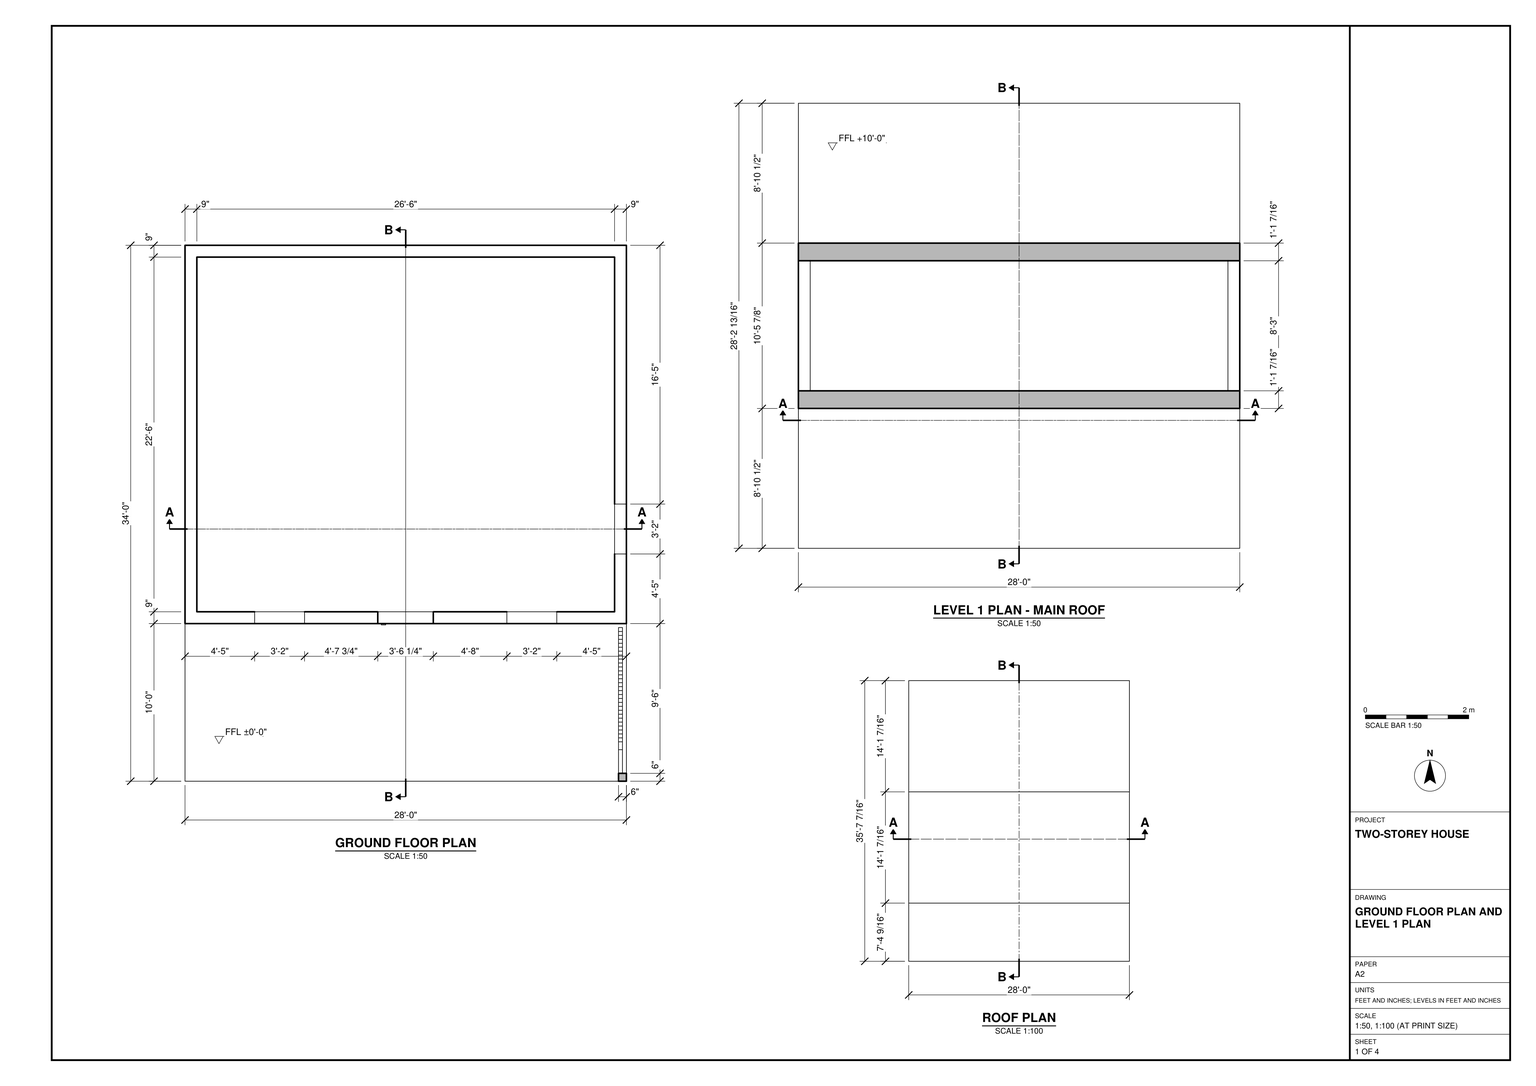
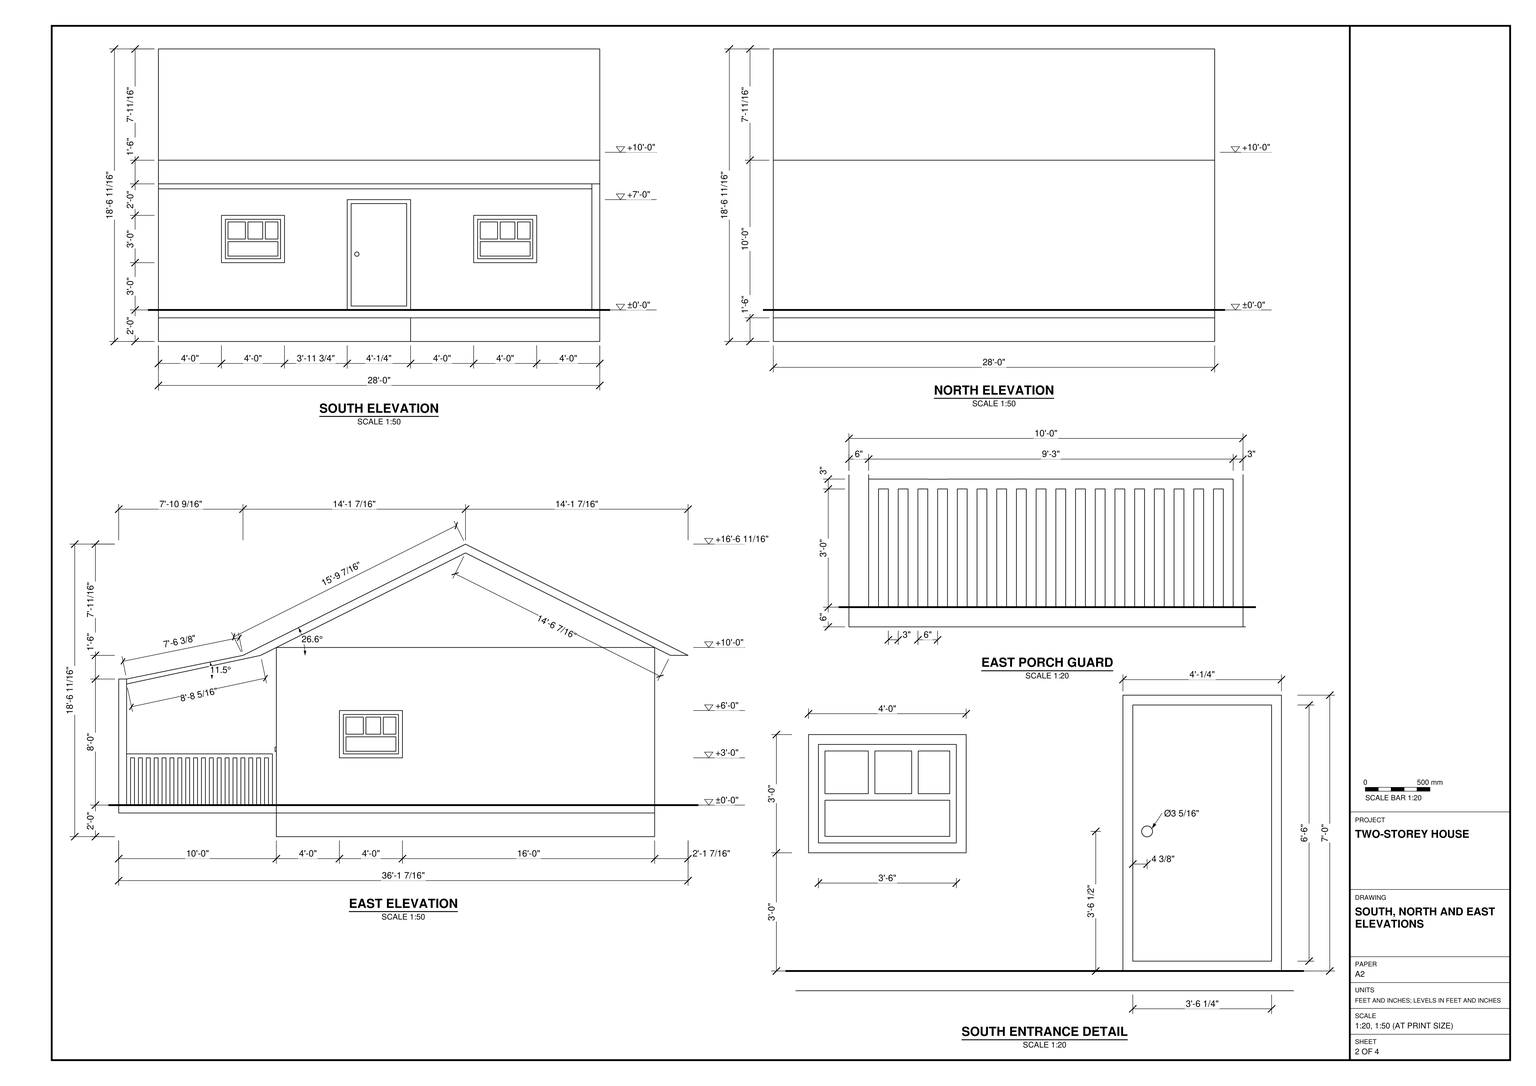
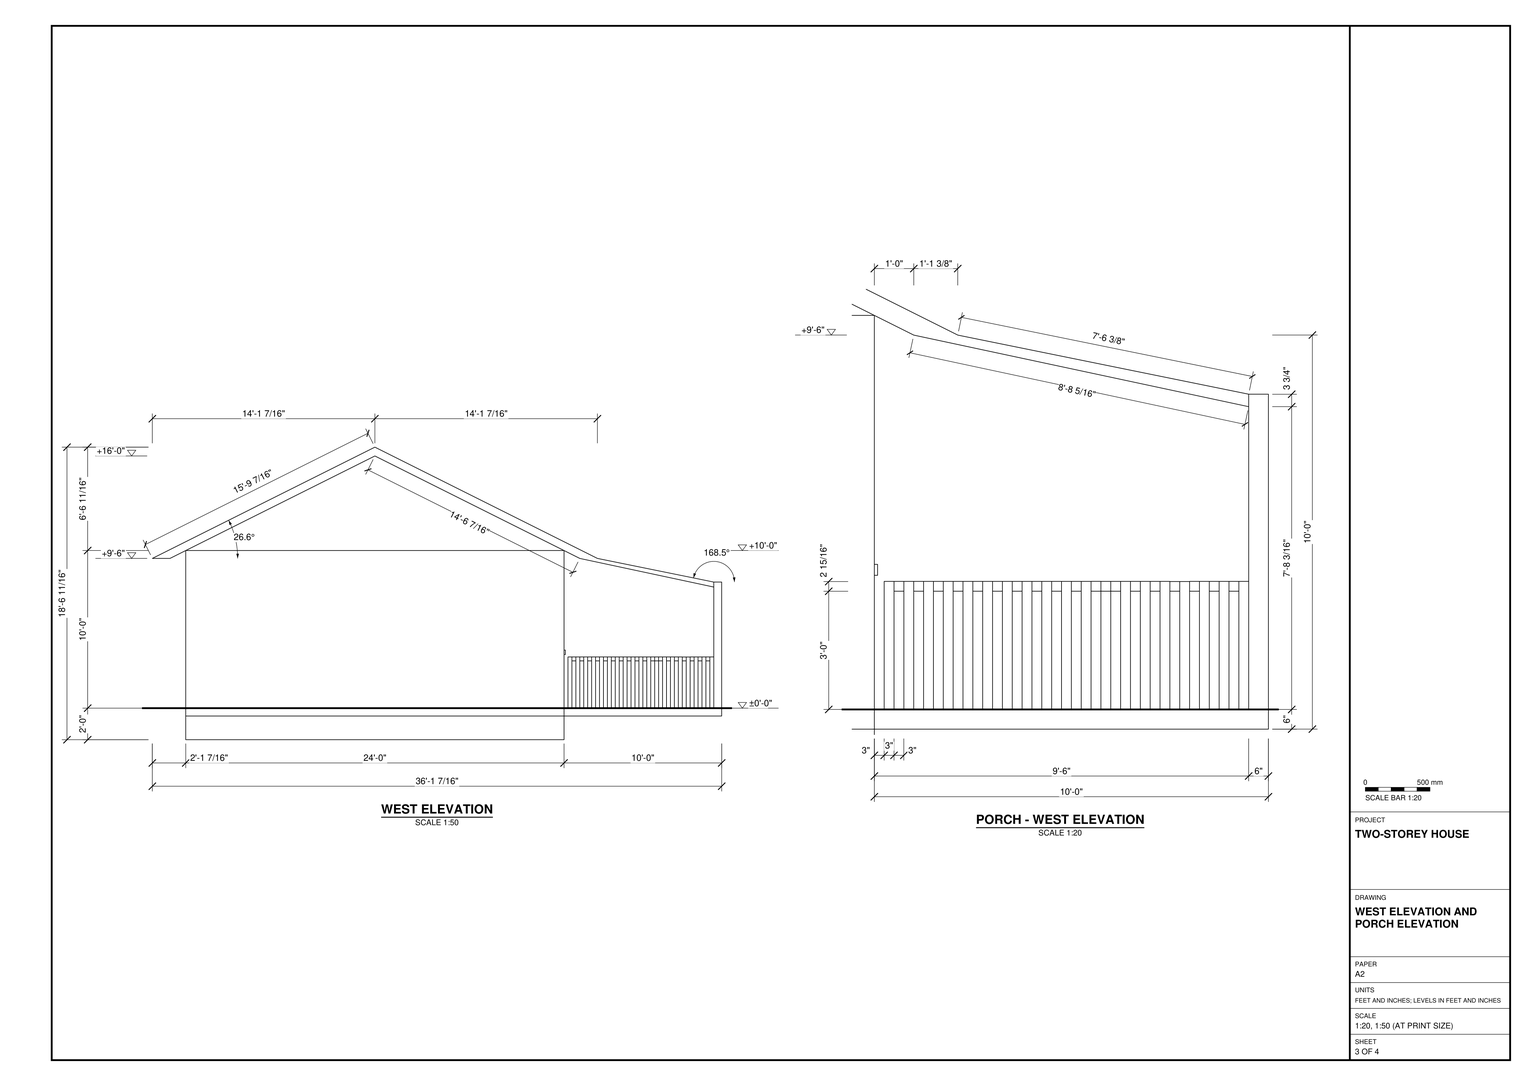
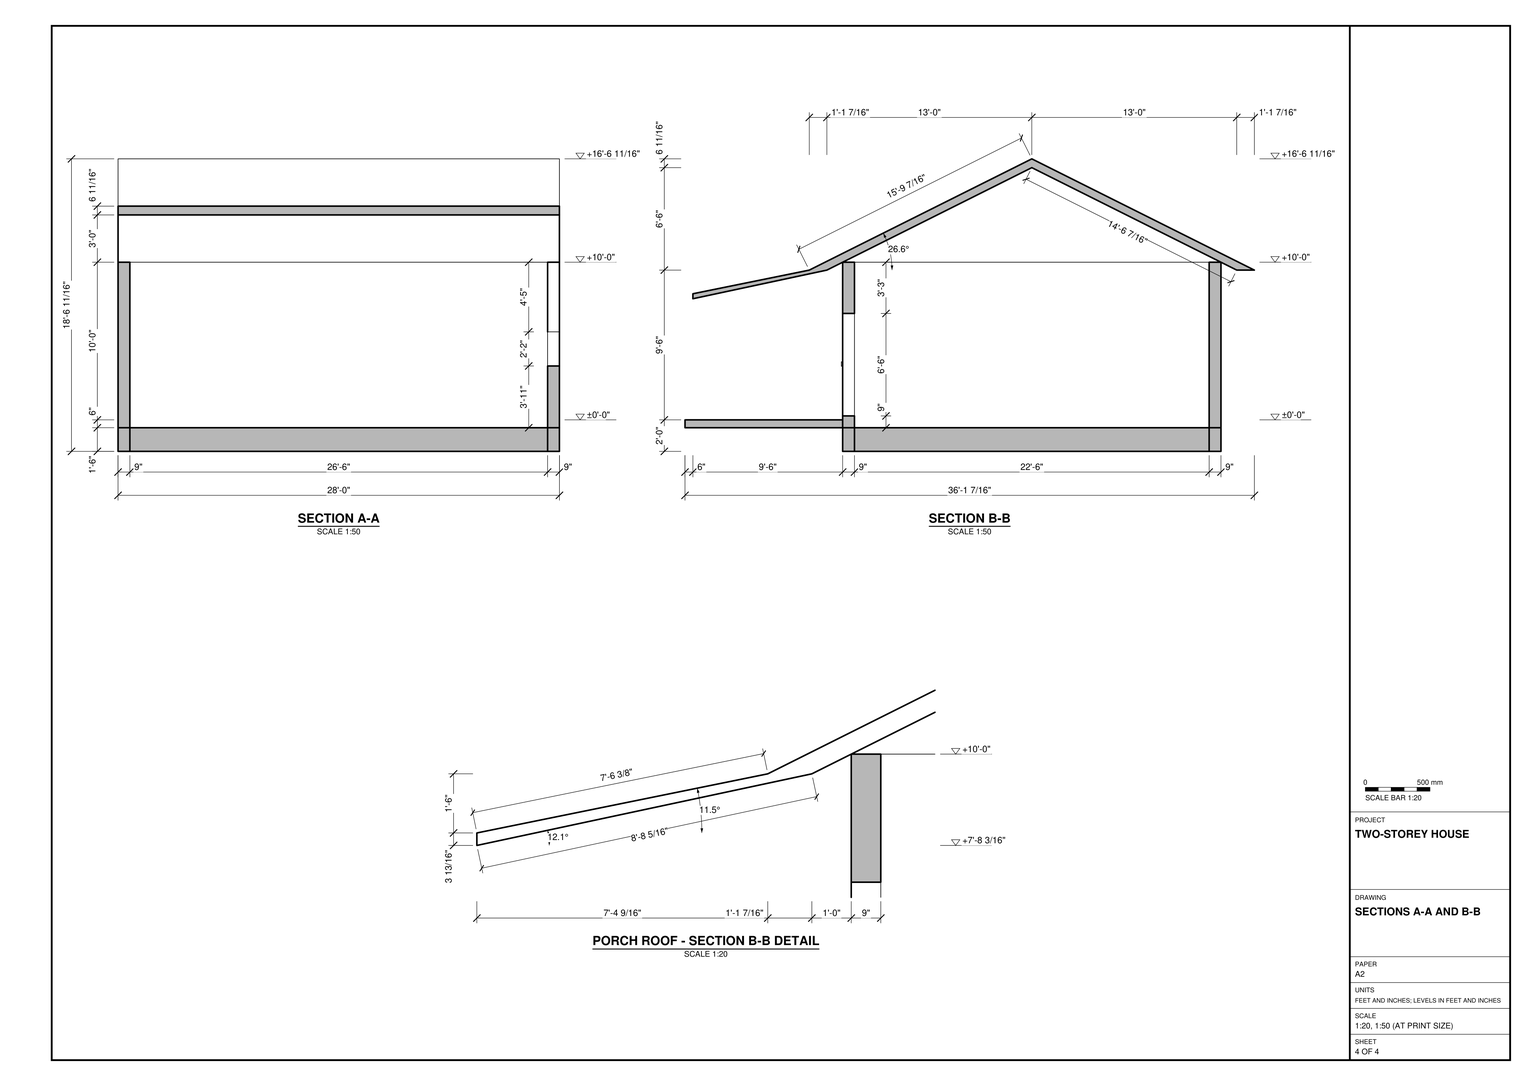
Build the house in SketchUp using task_files/diagram_01.pdf. Work in feet and inches. The overall model measures 28'-0" east to west, 36'-1 7/16" north to south and 18'-6 11/16" from the bottom of the base to the roof ridge. Set the ground floor at ±0'-0" and the main roof level at +10'-0".

Model the raised base, floor slab and rectangular enclosure with 9" exterior walls. Extend the floor across the full width of the south facade to form the 10'-0" deep porch. Use the plan to locate the entrance and window openings, and the elevation details to model the door leaf, frames and window pane divisions. Include the guard along the east edge of the porch and the roof support at its outer corner. Form the main roof with an east–west ridge. Give the roof its drawn thickness, carry the north slope beyond the rear wall and change to the shallower pitch over the porch.

Keep shell elements such as walls, slabs and roof separate as groups or components. Keep any furniture or joinery pieces separate in the same way, and use components for repeated parts. Decor and loose items may be any suitable library components. Save one SketchUp model as output_files/gable_roofed_house_with_a_covered_south_porch.skp.

# SketchUp Ruby script. Lengths in inches.
U = 1.inch
M = Sketchup.active_model
def pt(a) = Geom::Point3d.new(a.map { |v| v * U })
def face(e, loops, mat)
  f = e.add_face(loops[0].map { |a| pt(a) })
  loops[1..].each { |l| e.add_face(l.map { |a| pt(a) }).erase! }
  f.material = f.back_material = mat if mat
  f
end
# faces: each face lists its corners as indices into pts; further lists are holes
def faces(e, pts, list, mat = nil) = list.each { |f| face(e, (f[0].is_a?(Array) ? f : [f]).map { |l| l.map { |i| pts[i] } }, mat) }
# xy, xz, yz: faces in a plane at the given z, y or x. An outline is a flat list of corners, or four numbers for a rectangle; further outlines are holes
def ring(l) = l.size == 4 ? [[l[0], l[1]], [l[2], l[1]], [l[2], l[3]], [l[0], l[3]]] : l.each_slice(2).to_a
def flat(e, list, mat, &to3) = list.each { |f| face(e, (f[0].is_a?(Array) ? f : [f]).map { |l| ring(l).map { |u, v| to3.(u, v) } }, mat) }
def xy(e, z, list, mat = nil) = flat(e, list, mat) { |x, y| [x, y, z] }
def xz(e, y, list, mat = nil) = flat(e, list, mat) { |x, z| [x, y, z] }
def yz(e, x, list, mat = nil) = flat(e, list, mat) { |y, z| [x, y, z] }
def lines(e, pts, list) = list.each { |a, b| e.add_line(pt(pts[a]), pt(pts[b])) }
# prism: a flat outline (further loops are holes) pulled along v
def prism(e, loops, v, mat = nil)
  f = face(e, loops, mat); d = Geom::Vector3d.new(v.map { |x| x * U })
  f.pushpull(f.normal.samedirection?(d) ? d.length : -d.length)
end
def box(e, o, s, mat = nil) = prism(e, [[o, [o[0] + s[0], o[1], o[2]], [o[0] + s[0], o[1] + s[1], o[2]], [o[0], o[1] + s[1], o[2]]]], [0, 0, s[2]], mat)
def at(x, y, z, deg = 0) = Geom::Transformation.translation(pt([x, y, z])) * Geom::Transformation.rotation(ORIGIN, Z_AXIS, deg.degrees)
def axes(o, x, y, z) = Geom::Transformation.new([*x, 0, *y, 0, *z, 0, *pt(o).to_a, 1])
def part(name) = M.definitions.add(name)
# library, detail: a bought-in or finely detailed component or shape, given as its bounding box
def library(name, o, s) = part(name).tap { |d| box(d.entities, o, s) }
def detail(e, o, s) = box(e.add_group.entities, o, s)
def put(e, d, t, mat = nil) = e.add_instance(d, t).tap { |i| i.material = mat if mat }
def group(e, t, mat = nil) = e.add_group.tap { |g| g.transformation = t; g.material = mat if mat }.entities
root = M.entities
M.materials.add("Glass_Safety_01").color = [204, 235, 244]
M.materials["Glass_Safety_01"].alpha = 0.25
M.materials.add("I02_Moonlit_Azure").color = [153, 153, 255]
M.materials.add("Metal_06_1K").color = [238, 236, 231]
M.materials.add("Sree_Pearls_1").color = [252, 252, 252]
M.materials.add("Wood_Veneer_15_1K").color = [103, 69, 45]
xy(root,-24,[[[0,120,336,408],[9,129,327,399]],[9,129,327,399]])
xy(root,-6,[[0,0,336,120],[0,120,336,408]])
xy(root,0,[[[0,0,330,0,330,9,333,9,333,6,336,6,336,120,0,120],[330,12,333,15],[330,18,333,21],[330,24,333,27],[330,30,333,33],[330,36,333,39],[330,42,333,45],[330,48,333,51],[330,54,333,57],[330,60,333,63],[330,66,333,69],[330,72,333,75],[330,78,333,81],[330,84,333,87],[330,90,333,93],[330,96,333,99],[330,102,333,105],[330,108,333,111],[330,114,333,117]]])
xy(root,3,[[146.73,120,189,129]])
xy(root,36,[[330,9,333,12],[330,15,333,18],[330,21,333,24],[330,27,333,30],[330,33,333,36],
  [330,39,333,42],[330,57,333,60],[330,63,333,66],[330,69,333,72],[330,75,333,78],
  [330,81,333,84],[330,87,333,90],[330,93,333,96],[330,99,333,102],[330,105,333,108],
  [330,111,333,114]])
xy(root,38.95,[[330,24,333,27],[330,27,333,30]])
xy(root,39,[[330,6,333,24],[330,30,333,33],[330,33,333,36],[330,36,333,39],[330,39,333,42],
  [330,42,333,45],[330,45,333,48],[330,48,333,51],[330,54,333,57],[330,57,333,60],
  [330,60,333,63],[330,63,333,66],[330,66,333,69],[330,69,333,72],[330,72,333,75],
  [330,75,333,78],[330,78,333,81],[330,81,333,84],[330,84,333,87],[330,87,333,90],
  [330,90,333,93],[330,93,333,96],[330,96,333,99],[330,99,333,102],[330,102,333,105],
  [330,105,333,108],[330,108,333,111],[330,111,333,114],[330,114,333,117]])
xy(root,39.01,[[330,51,333,54]])
xy(root,41,[[53,120,91,129],[245,120,283,129],[327,173,336,211]])
xy(root,81,[[146.73,120,189,129]])
xy(root,96,[[330,0,336,6]])
xy(root,114,[[0,420,336,433.42]])
xy(root,120,[[[0,120,336,408],[9,129,327,399]]])
xz(root,0,[[0,-6,336,-6,336,96,330,96,330,0,0,0]])
xz(root,6,[[333,0,333,39,330,39,330,92.2,336,92.2,336,0],[330,92.2,336,96]])
xz(root,6,[[0,92.2,330,96]],"Sree_Pearls_1")
xz(root,9,[[330,0,333,36]])
xz(root,12,[[330,0,333,36]])
xz(root,15,[[330,0,333,36]])
xz(root,18,[[330,0,333,36]])
xz(root,21,[[330,0,333,36]])
xz(root,24,[[330,0,333,36],[330,38.95,333,39]])
xz(root,27,[[330,0,333,36]])
xz(root,30,[[330,0,333,36],[330,38.95,333,39]])
xz(root,33,[[330,0,333,36]])
xz(root,36,[[330,0,333,36]])
xz(root,39,[[330,0,333,36]])
xz(root,42,[[330,0,333,36]])
xz(root,45,[[330,0,333,36]])
xz(root,51,[[330,39,333,39.01]])
xz(root,54,[[330,0,333,36],[330,39,333,39.01]])
xz(root,57,[[330,0,333,36]])
xz(root,60,[[330,0,333,36]])
xz(root,63,[[330,0,333,36]])
xz(root,66,[[330,0,333,36]])
xz(root,69,[[330,0,333,36]])
xz(root,72,[[330,0,333,36]])
xz(root,75,[[330,0,333,36]])
xz(root,78,[[330,0,333,36]])
xz(root,81,[[330,0,333,36]])
xz(root,84,[[330,0,333,36]])
xz(root,87,[[330,0,333,36]])
xz(root,90,[[330,0,333,36]])
xz(root,93,[[330,0,333,36]])
xz(root,96,[[330,0,333,36]])
xz(root,99,[[330,0,333,36]])
xz(root,102,[[330,0,333,36]])
xz(root,105,[[330,0,333,36]])
xz(root,108,[[330,0,333,36]])
xz(root,111,[[330,0,333,36]])
xz(root,114,[[330,0,333,36]])
xz(root,117,[[330,0,333,39]])
xz(root,119,[[151.08,40.85,151.51,40.9,151.92,41.07,152.26,41.34,152.53,41.68,152.69,42.08,152.75,42.51,152.69,42.94,152.53,43.35,152.26,43.69,151.92,43.96,151.51,44.12,151.08,44.18,150.65,44.12,150.25,43.96,149.9,43.69,149.64,43.35,149.47,42.94,149.42,42.51,149.47,42.08,149.64,41.68,149.9,41.34,150.25,41.07,150.65,40.9]],"Metal_06_1K")
xz(root,120,[[0,-24,192,-6],[192,-24,336,-6],[0,-6,143.73,0],[143.73,-6,192,0],[192,-6,336,0],
  [[48,36,96,72],[51,39,93,69]],[[240,36,288,72],[243,39,285,69]],[[51,39,93,69],[53,41,91,52],[53,54,66.2,67],[68.2,54,79.4,67],[81.4,54,91,67]],[[243,39,285,69],[245,41,283,52],[245,54,258.2,67],[260.2,54,271.4,67],[273.4,54,283,67]]])
xz(root,120,[[53,41,91,52],[245,41,283,52],[53,54,66.2,67],[68.2,54,79.4,67],[81.4,54,91,67],
  [245,54,258.2,67],[260.2,54,271.4,67],[273.4,54,283,67]],"Glass_Safety_01")
xz(root,120,[[[0,0,143.73,0,143.73,84,192,84,192,0,336,0,336,120,0,120],[48,36,96,72],[240,36,288,72]]],"I02_Moonlit_Azure")
xz(root,120,[[[143.73,0,192,84],[146.73,3,189,81]],[[146.73,3,189,81],[151.08,40.85,150.65,40.9,150.25,41.07,149.9,41.34,149.64,41.68,149.47,42.08,149.42,42.51,149.47,42.94,149.64,43.35,149.9,43.69,150.25,43.96,150.65,44.12,151.08,44.18,151.51,44.12,151.92,43.96,152.26,43.69,152.53,43.35,152.69,42.94,152.75,42.51,152.69,42.08,152.53,41.68,152.26,41.34,151.92,41.07,151.51,40.9]]],"Wood_Veneer_15_1K")
xz(root,129,[[[9,-24,327,120],[146.73,3,189,81],[245,41,283,67],[53,41,91,67]]])
xz(root,399,[[9,-24,327,120]])
xz(root,408,[[0,-6,336,120]],"I02_Moonlit_Azure")
xz(root,408,[[0,-24,336,-6]],"Sree_Pearls_1")
yz(root,0,[[0,-6,120,0],[6,92.2,108,114,264,192,420,114,433.42,114,264,198.71,94.58,114,6,96]])
yz(root,0,[[120,-6,408,120],[120,120,264,192,408,120]],"I02_Moonlit_Azure")
yz(root,0,[[120,-24,408,-6]],"Sree_Pearls_1")
yz(root,9,[[129,-24,399,120]])
yz(root,146.73,[[120,3,129,81]])
yz(root,189,[[120,3,129,81]])
yz(root,327,[[[129,-24,399,120],[173,41,211,67]]])
yz(root,330,[[0,0,6,96],[6,0,9,39],[12,0,15,39],[18,0,21,39],[24,0,27,38.95],
  [30,0,33,39],[36,0,39,39],[42,0,45,39],[54,0,57,39],[60,0,63,39],
  [66,0,69,39],[72,0,75,39],[78,0,81,39],[84,0,87,39],[90,0,93,39],
  [96,0,99,39],[102,0,105,39],[108,0,111,39],[114,0,117,39],[9,36,12,39],
  [15,36,18,39],[21,36,24,39],[27,36,30,38.95],[33,36,36,39],[39,36,42,39],
  [45,36,48,39],[48,36,51,39],[51,36,54,39.01],[57,36,60,39],[63,36,66,39],
  [69,36,72,39],[75,36,78,39],[81,36,84,39],[87,36,90,39],[93,36,96,39],
  [99,36,102,39],[105,36,108,39],[111,36,114,39]])
yz(root,330,[[48,0,51,36]],"Sree_Pearls_1")
yz(root,333,[[6,0,9,0,9,36,12,36,12,0,15,0,15,36,18,36,18,0,21,0,21,36,24,36,24,0,27,0,27,36,30,36,30,0,33,0,33,36,36,36,36,0,39,0,39,36,42,36,42,0,45,0,45,36,48,36,48,0,51,0,51,36,54,36,54,0,57,0,57,36,60,36,60,0,63,0,63,36,66,36,66,0,69,0,69,36,72,36,72,0,75,0,75,36,78,36,78,0,81,0,81,36,84,36,84,0,87,0,87,36,90,36,90,0,93,0,93,36,96,36,96,0,99,0,99,36,102,36,102,0,105,0,105,36,108,36,108,0,111,0,111,36,114,36,114,0,117,0,117,39,54,39,54,39.01,51,39.01,51,39,30,39,30,38.95,24,38.95,24,39,6,39]])
yz(root,336,[[0,-6,120,-6,120,0,6,0,6,96,0,96],[[168,36,216,72],[171,39,213,69]],[[171,39,213,69],[173,41,211,52],[173,54,186.2,67],[188.2,54,199.4,67],[201.4,54,211,67]],[6,92.2,108,114,264,192,420,114,433.42,114,264,198.71,94.58,114,6,96]])
yz(root,336,[[173,41,211,52],[173,54,186.2,67],[188.2,54,199.4,67],[201.4,54,211,67]],"Glass_Safety_01")
yz(root,336,[[[120,-6,408,120],[168,36,216,72]],[120,120,408,120,264,192]],"I02_Moonlit_Azure")
yz(root,336,[[120,-24,408,-6]],"Sree_Pearls_1")
p = [[150.65,120,40.9],[151.08,120,40.85],[151.08,119,40.85],[150.65,119,40.9],[151.51,120,40.9],[151.51,119,40.9],
  [150.25,120,41.07],[150.25,119,41.07],[151.92,120,41.07],[151.92,119,41.07],[149.9,120,41.34],[149.9,119,41.34],
  [152.26,120,41.34],[152.26,119,41.34],[149.64,120,41.68],[149.64,119,41.68],[152.53,120,41.68],[152.53,119,41.68],
  [149.47,120,42.08],[149.47,119,42.08],[152.69,120,42.08],[152.69,119,42.08],[149.42,120,42.51],[149.42,119,42.51],
  [152.75,120,42.51],[152.75,119,42.51],[149.47,120,42.94],[149.47,119,42.94],[152.69,120,42.94],[152.69,119,42.94],
  [149.64,120,43.35],[149.64,119,43.35],[152.53,120,43.35],[152.53,119,43.35],[149.9,120,43.69],[149.9,119,43.69],
  [152.26,120,43.69],[152.26,119,43.69],[150.25,120,43.96],[150.25,119,43.96],[151.92,120,43.96],[151.92,119,43.96],
  [150.65,120,44.12],[150.65,119,44.12],[151.51,120,44.12],[151.51,119,44.12],[151.08,120,44.18],[151.08,119,44.18],
  [336,6,92.2],[336,108,114],[0,108,114],[0,6,92.2],[330,6,92.2],[336,94.58,114],
  [336,6,96],[330,6,96],[0,6,96],[0,94.58,114],[336,264,198.71],[0,264,198.71],
  [336,120,120],[0,120,120],[336,433.42,114],[0,433.42,114],[336,408,120],[336,420,114],
  [0,420,114],[0,408,120],[336,264,192],[0,264,192],[336,173,67],[327,173,67],
  [336,211,67],[327,211,67],[53,120,67],[53,129,67],[91,120,67],[91,129,67],
  [245,120,67],[245,129,67],[283,120,67],[283,129,67]]
faces(root,p,[[0,1,2,3],[1,4,5,2],[6,0,3,7],[4,8,9,5],[10,6,7,11],[8,12,13,9],[14,10,11,15],[12,16,17,13],
  [18,14,15,19],[16,20,21,17],[22,18,19,23],[20,24,25,21],[26,22,23,27],[24,28,29,25],[30,26,27,31],[28,32,33,29],
  [34,30,31,35],[32,36,37,33],[38,34,35,39],[36,40,41,37],[42,38,39,43],[40,44,45,41],[46,42,43,47],[44,46,47,45]],"Metal_06_1K")
faces(root,p,[[48,49,50,51,52],[49,60,61,50],[64,65,66,67],[60,68,69,61],[68,64,67,69]])
faces(root,p,[[53,54,55,56,57],[58,53,57,59],[62,58,59,63]],"Wood_Veneer_15_1K")
lines(root,p,[[70,71],[72,73],[74,75],[76,77],[78,79],[80,81]])
g1 = group(root,at(0,0,0),"Sree_Pearls_1")
xy(g1,0,[[0,0,336,120]])
